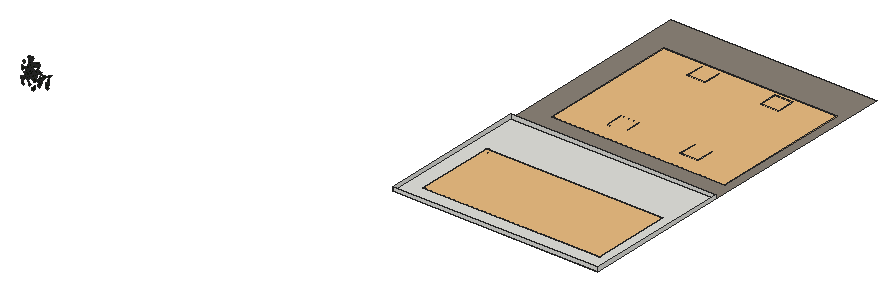
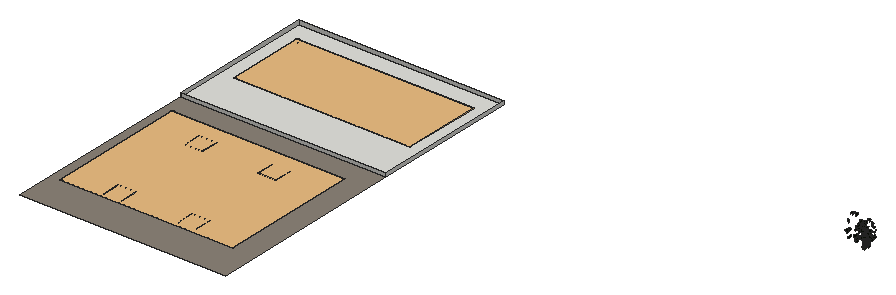
# SketchUp Ruby script. Lengths in inches.
U = 1.inch
M = Sketchup.active_model
def pt(a) = Geom::Point3d.new(a.map { |v| v * U })
def face(e, loops, mat)
  f = e.add_face(loops[0].map { |a| pt(a) })
  loops[1..].each { |l| e.add_face(l.map { |a| pt(a) }).erase! }
  f.material = f.back_material = mat if mat
  f
end
# faces: each face lists its corners as indices into pts; further lists are holes
def faces(e, pts, list, mat = nil) = list.each { |f| face(e, (f[0].is_a?(Array) ? f : [f]).map { |l| l.map { |i| pts[i] } }, mat) }
# xy, xz, yz: faces in a plane at the given z, y or x. An outline is a flat list of corners, or four numbers for a rectangle; further outlines are holes
def ring(l) = l.size == 4 ? [[l[0], l[1]], [l[2], l[1]], [l[2], l[3]], [l[0], l[3]]] : l.each_slice(2).to_a
def flat(e, list, mat, &to3) = list.each { |f| face(e, (f[0].is_a?(Array) ? f : [f]).map { |l| ring(l).map { |u, v| to3.(u, v) } }, mat) }
def xy(e, z, list, mat = nil) = flat(e, list, mat) { |x, y| [x, y, z] }
def xz(e, y, list, mat = nil) = flat(e, list, mat) { |x, z| [x, y, z] }
def yz(e, x, list, mat = nil) = flat(e, list, mat) { |y, z| [x, y, z] }
def lines(e, pts, list) = list.each { |a, b| e.add_line(pt(pts[a]), pt(pts[b])) }
# prism: a flat outline (further loops are holes) pulled along v
def prism(e, loops, v, mat = nil)
  f = face(e, loops, mat); d = Geom::Vector3d.new(v.map { |x| x * U })
  f.pushpull(f.normal.samedirection?(d) ? d.length : -d.length)
end
def box(e, o, s, mat = nil) = prism(e, [[o, [o[0] + s[0], o[1], o[2]], [o[0] + s[0], o[1] + s[1], o[2]], [o[0], o[1] + s[1], o[2]]]], [0, 0, s[2]], mat)
def at(x, y, z, deg = 0) = Geom::Transformation.translation(pt([x, y, z])) * Geom::Transformation.rotation(ORIGIN, Z_AXIS, deg.degrees)
def axes(o, x, y, z) = Geom::Transformation.new([*x, 0, *y, 0, *z, 0, *pt(o).to_a, 1])
def part(name) = M.definitions.add(name)
# library, detail: a bought-in or finely detailed component or shape, given as its bounding box
def library(name, o, s) = part(name).tap { |d| box(d.entities, o, s) }
def detail(e, o, s) = box(e.add_group.entities, o, s)
def put(e, d, t, mat = nil) = e.add_instance(d, t).tap { |i| i.material = mat if mat }
def group(e, t, mat = nil) = e.add_group.tap { |g| g.transformation = t; g.material = mat if mat }.entities
root = M.entities
M.materials.add("Heather_Band").color = [140, 131, 120]
M.materials.add("efeu1").color = [18, 25, 13]
M.materials.add("efeu2").color = [43, 57, 29]
c1 = part("ivyleaf_9")
p = [[1.54,2.16,1.25],[1.36,2.04,1.19],[-0.21,0.99,0.68],[-0.71,1.11,0.82],[-0.85,0.86,0.67],[-0.8,0.17,0.21],
  [-0.9,-0.01,0.1],[-0.67,-0.16,-0.02],[-0.08,-0.08,-0.05],[-0.03,-0.6,-0.4],[0.65,-0.88,-0.66],[0.83,-0.6,-0.49],
  [1.29,-0.42,-0.43],[1.8125,-0.07,-0.26],[1.21,0.44,0.15]]
faces(c1.entities,p,[[0,1,2,3,4,5,6,7,8,9,10,11,12,13,14]],"efeu1")
c2 = part("ivyleaf_10")
p = [[0,0.5,-0.03],[-0.0625,2.02,-0.43],[-0.19,2.01,-0.46],[-0.54,1.05,-0.29],[-0.52,0.625,-0.18],[-0.83,0.76,-0.28],
  [-1.16,0.64,-0.33],[-1.15,0.33,-0.24],[-0.77,-0.39,0.02],[-0.3,-0.51,0.16],[0.04,-0.48,0.23],[-0.02,2.01,-0.4375],
  [-0.06,2.01,-0.43],[0.04,-0.49,0.23],[0.67,-0.49,0.14],[1.38,0.36,-0.2],[1.375,0.51,-0.24],[0.81,0.65,-0.19],
  [0.62,0.59,-0.15],[0.6,1.09,-0.28],[0.5,1.23,-0.31]]
faces(c2.entities,p,[[0,1,2,3,4,5,6,7,8,9,10],[11,12,0,13,14,15,16,17,18,19,20]],"efeu2")
c3 = library("Tlon Light 450 Ceiling 152 006",[-8.86,-8.86,-3.78],[17.72,17.72,3.56])
c4 = part("Tlon Cubo 860 Ceiling 152 005")
xy(c4.entities,-3.04,[[-16.54,-16.54,-16.54,16.54,16.54,-16.54],[16.54,-16.54,-16.54,16.54,16.54,16.54]])
xy(c4.entities,0,[[-16.93,-16.93,16.93,-16.93,-16.93,16.93],[16.93,-16.93,16.93,16.93,-16.93,16.93]])
xz(c4.entities,-16.93,[[-16.93,-3.79,16.93,-3.79,-16.93,0],[16.93,-3.79,16.93,0,-16.93,0]])
xz(c4.entities,-16.3,[[-16.3,-3.66,-16.3,-3.24,16.3,-3.24],[-16.3,-3.66,16.3,-3.24,16.3,-3.66]])
xz(c4.entities,16.3,[[-16.3,-3.66,16.3,-3.24,-16.3,-3.24],[-16.3,-3.66,16.3,-3.66,16.3,-3.24]])
xz(c4.entities,16.93,[[-16.93,-3.79,-16.93,0,16.93,0],[-16.93,-3.79,16.93,0,16.93,-3.79]])
yz(c4.entities,-16.93,[[-16.93,-3.79,-16.93,0,16.93,0],[-16.93,-3.79,16.93,0,16.93,-3.79]])
yz(c4.entities,-16.3,[[-16.3,-3.66,16.3,-3.66,-16.3,-3.24],[16.3,-3.66,16.3,-3.24,-16.3,-3.24]])
yz(c4.entities,16.3,[[-16.3,-3.66,-16.3,-3.24,16.3,-3.66],[16.3,-3.66,-16.3,-3.24,16.3,-3.24]])
yz(c4.entities,16.93,[[-16.93,-3.79,16.93,-3.79,-16.93,0],[16.93,-3.79,16.93,0,-16.93,0]])
p = [[-16.93,-16.93,-3.79],[-16.93,16.93,-3.79],[-16.3,16.3,-3.66],[-16.3,-16.3,-3.66],[16.93,-16.93,-3.79],[16.3,-16.3,-3.66],
  [16.93,16.93,-3.79],[16.3,16.3,-3.66]]
faces(c4.entities,p,[[0,1,2],[2,3,0],[4,0,3],[3,5,4],[6,4,5],[5,7,6],[2,1,6],[6,7,2]])
c5 = library("Group\#12",[-0.5,-0.5,-0.1],[90.6875,40.6875,0.2])
c6 = library("Group\#6",[-0.5,-0.5,-0.1],[89,71.75,0.2])
xy(root,220.38,[[[233.9,233.25,339.25,308.9375],[242.26,243.41,331.94,283.1]],[244.26,245.41,329.94,281.1]])
xy(root,220.38,[[[233.9,308.9375,339.25,411.875],[246.39,320.92,334.39,391.67]],[248.39,322.92,332.39,389.67]],"Heather_Band")
xz(root,233.25,[[233.9,220.38,339.25,222.44]])
xz(root,308.9375,[[233.9,220.38,339.25,222.44]])
yz(root,233.9,[[233.25,220.38,308.9375,222.44]])
yz(root,339.25,[[233.25,220.38,308.9375,222.44]])
put(root,c1,axes([54.98,225.03,218.43],[-0.23169,-0.42688,-0.11871],[0.08282,0.08987,-0.48483],[0.43527,-0.24432,0.02907]))
put(root,c2,axes([55,225.69,216.45],[-0.00084,-0.39996,0.30006],[0.00049,0.30006,0.39996],[-0.5,0.00096,-0.00011]))
put(root,c1,axes([54.97,225.22,219.39],[0.33851,0.30535,0.20535],[0.06311,0.22671,-0.44116],[-0.36253,0.3246,0.11494]))
put(root,c2,axes([55.02,224.84,220.64],[-0.115,0.48191,0.06734],[-0.00438,0.06816,-0.49531],[-0.48658,-0.11451,-0.01145]))
put(root,c2,axes([55.18,225.16,220.32],[-0.13194,0.22964,0.42409],[-0.20569,0.37089,-0.26483],[-0.43621,-0.24435,-0.0034]))
put(root,c2,axes([55.07,222.89,215.11],[0.40029,-0.29956,-0.00596],[-0.00291,0.00605,-0.49995],[0.2996,0.40028,0.0031]))
put(root,c2,axes([55.2,225.59,215.35],[-0.48941,0.05551,0.08603],[-0.09025,-0.03545,-0.49051],[-0.04836,-0.49564,0.04472]))
put(root,c2,axes([55.1,225.36,218.1875],[0.4411,0.21357,-0.09907],[-0.11912,0.02098,-0.48515],[-0.20307,0.4516,0.06939]))
put(root,c1,axes([55.35,223.37,219.42],[-0.00289,-0.02393,-0.49942],[-0.18865,-0.46246,0.02325],[-0.46303,0.18857,-0.00636]))
put(root,c2,axes([55.17,225.84,215.27],[-0.33164,-0.37393,-0.01363],[0.00896,0.01027,-0.49981],[0.37407,-0.33176,-0.00011]))
put(root,c1,axes([54.9,225.19,217.71],[0.12618,-0.43294,-0.21595],[0.00232,0.22372,-0.44715],[0.48381,0.11185,0.05847]))
put(root,c2,axes([55.06,225.375,217.07],[-0.09279,0.48792,-0.05762],[0.004,-0.05789,-0.49662],[-0.4913,-0.09262,0.00684]))
put(root,c2,axes([55.1,225.22,218.61],[0.04069,0.4722,0.15929],[-0.06853,0.1636,-0.46748],[-0.49361,0.01621,0.07804]))
put(root,c2,axes([55.11,225.46,215.25],[0.48874,0.07712,-0.07203],[-0.07758,0.03125,-0.49296],[-0.07154,0.49303,0.04251]))
put(root,c1,axes([54.91,224.89,221.14],[0.04748,-0.45209,0.20822],[0.06666,-0.20151,-0.45272],[0.49326,0.07075,0.04114]))
put(root,c2,axes([55.06,225.64,214.14],[0.42748,0.2575,-0.03091],[-0.02865,-0.01234,-0.49903],[-0.25777,0.42841,0.0042]))
put(root,c2,axes([55.48,225.55,217.93],[-0.02537,-0.02326,0.49881],[-0.44758,-0.22041,-0.03304],[0.22142,-0.4482,-0.00964]))
put(root,c2,axes([55.13,225.61,215.41],[0.11345,-0.48115,0.07502],[0.04011,-0.06753,-0.49379],[0.4853,0.11806,0.02328]))
put(root,c1,axes([55.14,222.93,215.22],[0.37667,0.26283,-0.19759],[-0.16609,-0.10724,-0.45925],[-0.28379,0.41161,0.00652]))
put(root,c1,axes([54.97,221.875,218.92],[0.47979,-0.04843,-0.13211],[-0.12845,0.0409,-0.48148],[0.05744,0.49597,0.02681]))
put(root,c1,axes([55.03,224.45,223.09],[-0.13546,-0.46558,0.122],[0.01544,-0.13088,-0.48232],[0.48105,-0.12691,0.04983]))
put(root,c2,axes([55.1,222.73,216.23],[0.09381,-0.47349,0.13041],[0.08738,-0.11456,-0.47879],[0.48329,0.11262,0.06125]))
put(root,c2,axes([55.1875,225.19,219.27],[-0.49454,-0.07334,0.00706],[0.00901,-0.10771,-0.48818],[0.07313,-0.48272,0.10786]))
put(root,c2,axes([54.95,225.1,217.73],[0.44122,0.10916,0.20835],[0.15361,0.20166,-0.43097],[-0.17812,0.44431,0.14442]))
put(root,c2,axes([55.07,225.18,217.88],[-0.3955,-0.24587,-0.18201],[0.1889,0.0377,-0.4614],[0.24061,-0.43374,0.06307]))
put(root,c1,axes([54.97,222.98,214.22],[0.01627,0.22192,-0.44776],[0.03659,0.44626,0.22251],[0.49839,-0.04001,-0.00172]))
put(root,c2,axes([55.11,224.94,220.11],[0.43442,-0.24623,0.02552],[0.03209,0.00492,-0.49894],[0.24546,0.43514,0.02008]))
put(root,c2,axes([55.14,224.79,221.33],[-0.19138,0.46167,0.0154],[-0.00341,0.01526,-0.49976],[-0.46191,-0.19139,-0.00269]))
put(root,c1,axes([54.93,222.7,214.04],[-0.01095,-0.00019,-0.49988],[0.47255,-0.16305,-0.01029],[-0.16301,-0.47267,0.00375]))
put(root,c2,axes([55.16,224.19,215.49],[0.34017,-0.36405,0.04181],[0.02779,-0.03126,-0.49825],[0.36539,0.3413,-0.00104]))
put(root,c1,axes([54.9,222.3,217.9375],[0.1331,0.27101,-0.39855],[0.14321,0.37255,0.30116],[0.46019,-0.19432,0.02155]))
put(root,c2,axes([55.18,225.73,214.67],[0.06126,0.48896,-0.08463],[-0.06291,-0.07693,-0.49002],[-0.49223,0.07069,0.05209]))
put(root,c1,axes([55.26,225.16,219.31],[0.20578,0.45538,-0.01686],[-0.0094,-0.01425,-0.49971],[-0.45559,0.20598,0.0027]))
put(root,c2,axes([55.15,222.92,215.3],[-0.4769,-0.02322,-0.14842],[0.15018,-0.08451,-0.46936],[-0.00329,-0.49226,0.08758]))
put(root,c2,axes([55.4,223.25,216.93],[-0.36348,-0.27824,0.20117],[-0.15567,-0.12756,-0.4577],[0.30602,-0.39536,0.0061]))
put(root,c2,axes([55.17,223.98,217.33],[-0.11658,0.48613,0.00937],[-0.00028,0.00957,-0.49991],[-0.48622,-0.11656,-0.00196]))
put(root,c2,axes([55.1875,225.45,217.25],[-0.09419,0.49076,0.01675],[-0.02143,0.01293,-0.49937],[-0.49058,-0.09479,0.0186]))
put(root,c1,axes([54.86,221.46,216.96],[0.1271,-0.133,0.46493],[0.3745,-0.27706,-0.18163],[0.30593,0.3944,0.02919]))
put(root,c1,axes([55.03,223.78,217.11],[0.32284,-0.30897,-0.2243],[-0.05354,0.2542,-0.42722],[0.37803,0.29986,0.13105]))
put(root,c2,axes([55.1,225.47,216.09],[-0.36932,-0.14898,-0.30233],[0.29128,0.08456,-0.3975],[0.16957,-0.46974,0.02433]))
put(root,c2,axes([55.36,224.05,216.09],[-0.28204,-0.41122,0.03678],[-0.02073,-0.03038,-0.49865],[0.41234,-0.2828,0.00009]))
put(root,c2,axes([55.18,225.79,214.73],[0.37378,-0.30659,0.12764],[0.10332,-0.07528,-0.48338],[0.31562,0.38773,0.00707]))
put(root,c1,axes([55.13,219.31,216.17],[-0.02225,-0.462,-0.18989],[0.00751,0.18975,-0.46254],[0.49945,-0.02344,-0.00151]))
put(root,c2,axes([55.65,223.27,214.67],[-0.14566,-0.01431,0.4781],[-0.43865,-0.19526,-0.13949],[0.1907,-0.46007,0.04433]))
put(root,c2,axes([55.16,225.52,215.9375],[0.24012,-0.30822,0.312],[0.20942,-0.23195,-0.39031],[0.38534,0.31812,0.0177]))
put(root,c2,axes([55.125,225.06,220.29],[0.47221,0.04717,0.15746],[0.15244,0.05347,-0.47318],[-0.06148,0.49489,0.03612]))
put(root,c2,axes([55.6875,224.08,217.53],[-0.01704,0.49807,0.04049],[-0.49951,-0.01812,0.01262],[0.01404,-0.04002,0.4982]))
put(root,c2,axes([55.26,225.83,215],[0.31703,0.38311,-0.05215],[-0.03529,-0.03849,-0.49727],[-0.38503,0.31898,0.00264]))
put(root,c2,axes([55.36,225.73,215.62],[-0.35128,0.35297,0.04491],[-0.02724,0.03624,-0.49794],[-0.35477,-0.35228,-0.00623]))
put(root,c2,axes([55.38,225.53,216.51],[0.49365,0.06359,-0.04761],[-0.049,0.0079,-0.49753],[-0.06252,0.49588,0.01403]))
put(root,c1,axes([55.75,223.75,216.55],[-0.07628,0.49414,0.00225],[-0.49395,-0.07631,0.01366],[0.01384,-0.00014,0.49981]))
put(root,c2,axes([55.43,224.02,215.46],[-0.48754,0.10448,-0.0373],[0.03616,-0.00927,-0.4986],[-0.10488,-0.48887,0.00148]))
put(root,c1,axes([55.16,224.65,222.3],[0.30771,-0.39049,0.05327],[0.02443,-0.04855,-0.49704],[0.39335,0.30848,-0.0108]))
put(root,c2,axes([55.09,223.37,214.24],[0.02115,-0.07373,0.49408],[0.49436,-0.06802,-0.03131],[0.07183,0.48983,0.07002]))
put(root,c2,axes([55.17,220.11,222.98],[-0.1968,0.13634,-0.43895],[0.37732,-0.22476,-0.23898],[-0.26248,-0.42532,-0.01442]))
put(root,c1,axes([55.7,225.66,217.87],[-0.05507,0.22805,0.44154],[-0.09521,0.43117,-0.23457],[-0.48775,-0.10992,-0.00407]))
put(root,c2,axes([55.23,223.95,221.65],[0.16885,-0.15668,0.44378],[0.34407,-0.28059,-0.22997],[0.3211,0.38304,0.01306]))
put(root,c1,axes([55.44,220.16,215.7],[-0.06018,0.24632,-0.43093],[-0.11129,0.41634,0.25353],[0.48373,0.12643,0.00472]))
put(root,c1,axes([55.48,221.6875,216.93],[0.19435,-0.38004,-0.26038],[0.13203,-0.22479,0.42666],[-0.44136,-0.2346,0.01298]))
put(root,c1,axes([55.34,224.61,222.87],[0.47406,0.15311,0.04268],[0.04165,0.00992,-0.49816],[-0.15339,0.47588,-0.00335]))
put(root,c1,axes([55.84,223.7,222.27],[-0.38315,0.31909,0.03712],[-0.02852,0.02375,-0.49862],[-0.31997,-0.38421,0]))
put(root,c2,axes([55.98,223.16,214.74],[-0.15936,-0.00835,0.47385],[-0.47334,-0.02196,-0.15958],[0.02348,-0.49945,-0.0009]))
put(root,c1,axes([55.41,223.59,216.92],[0.45631,0.0971,0.17986],[0.171,0.05968,-0.46604],[-0.11197,0.48684,0.02126]))
put(root,c1,axes([56.03,218.875,220.56],[-0.47569,-0.04838,-0.14623],[-0.14557,-0.01391,0.47814],[-0.05033,0.49746,-0.00085]))
put(root,c1,axes([55.58,223.9,219.16],[-0.29351,-0.12273,-0.38573],[0.35326,0.15498,-0.3181],[0.19765,-0.45926,-0.00426]))
put(root,c2,axes([55.43,223.83,216.74],[0.13747,0.01167,0.48059],[0.46222,0.13415,-0.13548],[-0.1321,0.48153,0.02609]))
put(root,c1,axes([55.73,223.3,221.22],[0.07107,0.44434,-0.21796],[0.01792,0.21775,0.44974],[0.4946,-0.07174,0.01503]))
put(root,c1,axes([56.13,225.99,218.46],[0.03568,0.21012,0.4523],[0.06247,0.448,-0.21305],[-0.4948,0.07171,0.00571]))
put(root,c2,axes([56.44,223.38,220.95],[-0.06236,0.06455,-0.49188],[-0.43324,0.23444,0.08569],[0.24169,0.43689,0.0267]))
put(root,c1,axes([56.22,223.15,216.13],[-0.02852,-0.07705,-0.4932],[0.48784,0.10044,-0.0439],[0.10584,-0.48371,0.06945]))
put(root,c1,axes([56.71,223.2,216.98],[-0.2655,0.39663,-0.14898],[-0.08283,0.12383,0.47729],[0.41551,0.27812,-0.00005]))
put(root,c1,axes([56.45,216.85,217.61],[0.30055,-0.39778,0.03794],[0.02554,-0.02825,-0.49855],[0.39877,0.30162,0.00334]))
put(root,c1,axes([56.74,226.31,219.22],[0.29084,-0.16312,-0.37256],[-0.32628,0.17985,-0.33346],[0.2428,0.43709,-0.00183]))
put(root,c1,axes([56.74,217.02,215.43],[0.37439,-0.17131,-0.28369],[-0.25677,0.12065,-0.41172],[0.20952,0.45398,0.00236]))
put(root,c1,axes([56.84,221.22,216.58],[-0.42614,-0.13319,-0.22509],[0.21822,0.05613,-0.44635],[0.14417,-0.47865,0.01029]))
put(root,c1,axes([57.12,219.24,218.42],[0.05972,-0.07686,-0.49043],[-0.13411,0.47311,-0.09047],[0.47796,0.14235,0.0359]))
put(root,c1,axes([57.22,221.67,218.54],[0.3137,0.2943,0.25491],[0.18393,0.17651,-0.43013],[-0.34316,0.36364,0.00248]))
put(root,c1,axes([57.58,218.6,217.57],[0.05742,0.08209,-0.48986],[0.30213,0.38563,0.10004],[0.39424,-0.30749,-0.00531]))
put(root,c1,axes([57.95,222.1,216.48],[-0.0162,-0.11308,-0.48678],[0.00188,0.48701,-0.1132],[0.49973,-0.0055,-0.01536]))
put(root,c1,axes([57.875,223.375,220.08],[0.36514,0.22384,0.25801],[0.21173,0.14805,-0.42808],[-0.26804,0.42187,0.01333]))
put(root,c1,axes([58.29,221.75,218.18],[0.19494,0.38635,-0.25047],[0.09923,0.23035,0.43254],[0.44961,-0.21835,0.01313]))
put(root,c1,axes([58.6,220.05,222.2],[0.02983,0.07413,0.49357],[-0.16995,-0.4634,0.07987],[0.46928,-0.17253,-0.00245]))
put(root,c1,axes([59,223.23,222.15],[0.43873,-0.22893,0.07148],[0.06182,-0.03603,-0.49485],[0.23172,0.44305,-0.00332]))
put(root,c1,axes([59.59,223.15,221.94],[-0.00986,-0.0651,-0.49565],[0.01194,0.49557,-0.06533],[0.49976,-0.01313,-0.00821]))
put(root,c1,axes([60.23,219.36,219.21],[-0.14979,0.22131,-0.4226],[-0.32451,0.27739,0.26029],[0.34965,0.35225,0.06054]))
put(root,c1,axes([60.42,217.42,215.15],[0.08539,-0.13608,0.47349],[-0.25403,0.39957,0.16065],[-0.42211,-0.268,-0.0009]))
put(root,c1,axes([60,222.83,218.9375],[-0.22535,-0.05988,-0.4423],[0.43639,0.07448,-0.23242],[0.09372,-0.49078,0.01869]))
put(root,c1,axes([60.5,222.26,220.29],[0.07825,0.34131,0.35691],[0.06543,0.35101,-0.35001],[-0.48948,0.10149,0.01027]))
put(root,c1,axes([60.49,216.02,221.19],[-0.42877,-0.21341,-0.14356],[0.1286,0.06381,-0.47895],[0.22275,-0.44764,0.00016]))
put(root,c1,axes([60.16,221.57,222.28],[0.06104,-0.2281,0.44073],[0.2015,-0.39441,-0.23203],[0.45351,0.20594,0.04377]))
put(root,c1,axes([60.39,218.12,219.98],[0.11565,0.45517,0.1716],[-0.06521,-0.16029,0.4691],[0.48205,-0.13088,0.02229]))
put(root,c1,axes([60.77,222.88,220.91],[-0.3391,0.30234,-0.2088],[0.13849,-0.158,-0.45371],[-0.34034,-0.36554,0.02341]))
put(root,c1,axes([60.92,223.2,214.2],[-0.09936,-0.47899,0.10345],[-0.02375,-0.10072,-0.48917],[0.48945,-0.10212,-0.00273]))
put(root,c1,axes([61.3125,222.25,215.4],[0.03018,-0.04454,-0.4971],[-0.33033,0.37153,-0.05335],[0.37413,0.33163,-0.007]))
put(root,c1,axes([61.68,223.09,215.85],[0.27591,0.11303,0.40137],[-0.36894,-0.15812,0.29813],[0.19433,-0.46068,-0.00385]))
put(root,c1,axes([61.47,223.12,214.35],[-0.04807,0.04005,0.49607],[0.27085,-0.41601,0.05984],[0.41753,0.27447,0.0183]))
put(root,c1,axes([61.82,219.49,219.37],[-0.05344,-0.18906,0.45978],[-0.05097,-0.45791,-0.19421],[0.49452,-0.06763,0.02967]))
put(root,c1,axes([61.85,219.38,220.82],[-0.00312,0.02422,-0.4994],[0.30709,0.39421,0.0172],[0.39457,-0.30662,-0.01734]))
put(root,c1,axes([61.96,222.27,218.8],[0.44335,-0.13008,-0.19109],[0.18537,-0.04688,0.462],[-0.13811,-0.4805,0.00665]))
put(root,c1,axes([62.3,217.1875,213.73],[-0.25042,-0.14083,0.40922],[0.34686,0.21743,0.28708],[-0.25881,0.42766,-0.0112]))
put(root,c1,axes([62.17,219.48,219.94],[-0.2472,-0.13698,-0.41247],[0.38086,0.16032,-0.2815],[0.20937,-0.45336,0.02509]))
put(root,c1,axes([62.91,217.77,217.92],[-0.14574,0.02832,0.47745],[-0.46955,0.08649,-0.14846],[-0.091,-0.49165,0.00138]))
put(root,c1,axes([62.39,221.18,214.93],[0.27101,-0.34907,-0.2339],[-0.14252,0.18546,-0.44192],[0.39528,0.3062,0.00103]))
put(root,c1,axes([65.0625,217.5625,216.05],[0.31542,-0.37591,-0.09591],[0.06527,-0.07043,0.49069],[-0.38243,-0.32207,0.00464]))
put(root,c1,axes([65.36,222.64,214.12],[-0.2636,-0.3981,0.14843],[0.08158,0.124,0.47746],[-0.41697,0.27593,-0.00042]))
put(root,c1,axes([65.07,223.8,217.69],[0.12564,0.37158,-0.31007],[0.09396,0.29552,0.39222],[0.47475,-0.15683,0.00444]))
put(root,c1,axes([65.29,217.55,222.21],[0.02679,-0.0044,0.49926],[0.35813,-0.3482,-0.02229],[0.34789,0.3588,-0.0155]))
put(root,c1,axes([67.63,219.17,215.75],[0.43464,0.15735,-0.1906],[-0.17984,-0.06316,-0.46224],[-0.16955,0.47037,0.0017]))
put(root,c1,axes([68.4,216.99,221.88],[-0.33206,-0.36763,-0.06771],[0.04669,0.04907,-0.49539],[0.37088,-0.33533,0.00174]))
put(root,c1,axes([68.33,219.23,219.2],[-0.07433,-0.06032,-0.49075],[0.49039,0.05446,-0.08097],[0.06322,-0.49335,0.05107]))
put(root,c3,axes([262.11,254.77,218.57],[0.462,0,0],[0,0.462,0],[0,0,0.462]))
put(root,c4,axes([271.62,333.79,220.38],[0.2697,0,0],[0,0.2697,0],[0,0,0.2697]))
put(root,c4,axes([271.62,385.41,220.38],[0.2697,0,0],[0,0.2697,0],[0,0,0.2697]))
put(root,c5,at(242.26,243.41,220.38))
put(root,c6,at(246.39,320.92,220.38))
put(root,c4,axes([309.24,333.79,220.38],[0.2697,0,0],[0,0.2697,0],[0,0,0.2697]))
put(root,c4,axes([309.24,385.41,220.38],[0.2697,0,0],[0,0.2697,0],[0,0,0.2697]))
put(root,c3,axes([313.61,254.77,218.57],[0.462,0,0],[0,0.462,0],[0,0,0.462]))
